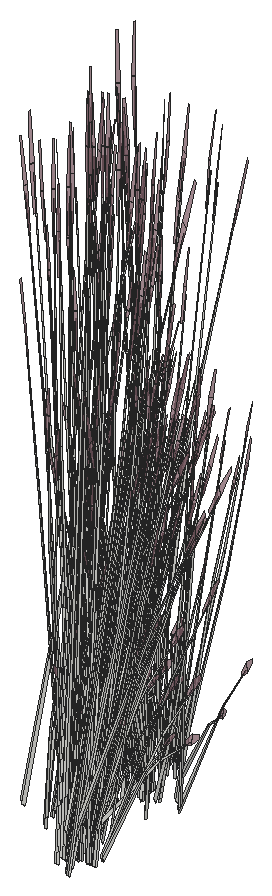
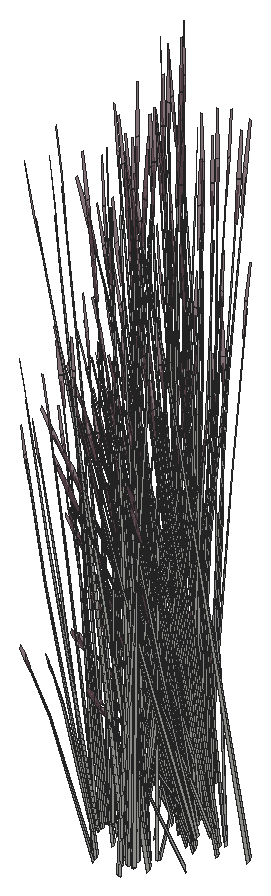
# SketchUp Ruby script. Lengths in inches.
U = 1.inch
M = Sketchup.active_model
def pt(a) = Geom::Point3d.new(a.map { |v| v * U })
def face(e, loops, mat)
  f = e.add_face(loops[0].map { |a| pt(a) })
  loops[1..].each { |l| e.add_face(l.map { |a| pt(a) }).erase! }
  f.material = f.back_material = mat if mat
  f
end
# faces: each face lists its corners as indices into pts; further lists are holes
def faces(e, pts, list, mat = nil) = list.each { |f| face(e, (f[0].is_a?(Array) ? f : [f]).map { |l| l.map { |i| pts[i] } }, mat) }
# xy, xz, yz: faces in a plane at the given z, y or x. An outline is a flat list of corners, or four numbers for a rectangle; further outlines are holes
def ring(l) = l.size == 4 ? [[l[0], l[1]], [l[2], l[1]], [l[2], l[3]], [l[0], l[3]]] : l.each_slice(2).to_a
def flat(e, list, mat, &to3) = list.each { |f| face(e, (f[0].is_a?(Array) ? f : [f]).map { |l| ring(l).map { |u, v| to3.(u, v) } }, mat) }
def xy(e, z, list, mat = nil) = flat(e, list, mat) { |x, y| [x, y, z] }
def xz(e, y, list, mat = nil) = flat(e, list, mat) { |x, z| [x, y, z] }
def yz(e, x, list, mat = nil) = flat(e, list, mat) { |y, z| [x, y, z] }
def lines(e, pts, list) = list.each { |a, b| e.add_line(pt(pts[a]), pt(pts[b])) }
# prism: a flat outline (further loops are holes) pulled along v
def prism(e, loops, v, mat = nil)
  f = face(e, loops, mat); d = Geom::Vector3d.new(v.map { |x| x * U })
  f.pushpull(f.normal.samedirection?(d) ? d.length : -d.length)
end
def box(e, o, s, mat = nil) = prism(e, [[o, [o[0] + s[0], o[1], o[2]], [o[0] + s[0], o[1] + s[1], o[2]], [o[0], o[1] + s[1], o[2]]]], [0, 0, s[2]], mat)
def at(x, y, z, deg = 0) = Geom::Transformation.translation(pt([x, y, z])) * Geom::Transformation.rotation(ORIGIN, Z_AXIS, deg.degrees)
def axes(o, x, y, z) = Geom::Transformation.new([*x, 0, *y, 0, *z, 0, *pt(o).to_a, 1])
def part(name) = M.definitions.add(name)
# library, detail: a bought-in or finely detailed component or shape, given as its bounding box
def library(name, o, s) = part(name).tap { |d| box(d.entities, o, s) }
def detail(e, o, s) = box(e.add_group.entities, o, s)
def put(e, d, t, mat = nil) = e.add_instance(d, t).tap { |i| i.material = mat if mat }
def group(e, t, mat = nil) = e.add_group.tap { |g| g.transformation = t; g.material = mat if mat }.entities
root = M.entities
M.materials.add("LightPink_Translucent").color = [144, 107, 117]
M.materials["LightPink_Translucent"].alpha = 0.75
c1 = part("blade")
p = [[2.15,0.21,22],[0,0.17,0],[0.09,0.45,0],[2.18,0.31,22],[2.29,0.31,22],[0.38,0.45,0],
  [2.48,0.24,33],[2.49,0.24,33],[2.48,0.22,33]]
faces(c1.entities,p,[[0,1,2,3],[4,5,2,3],[6,3,4,7],[8,0,3,6]])
c2 = part("seeds")
p = [[0.3,-0.1,1.38],[-0.01,-0.03,1.59],[-0.01,-0.03,0.03],[0.14,-0.07,-0.07],[0.29,-0.03,3],[0.15,0.01,3.11]]
faces(c2.entities,p,[[0,1,2,3],[1,0,4,5]],"LightPink_Translucent")
c3 = part("blade with seeds")
put(c3.entities,c1,at(0,0,0))
put(c3.entities,c2,axes([2.4,0.25,30.99],[1.5799,-0.05474,1.17369],[-0.12525,1.92788,0.29478],[-0.07173,-0.02425,1.56792]))
put(root,c3,axes([411.99,41.31,-7.78],[0.42502,0.15163,-0.32977],[-0.12396,0.44238,0.42575],[0.17112,-0.04056,0.81462]))
put(root,c3,axes([411.24,39.4,-10.12],[0.47863,0.27177,-0.46235],[-0.28609,0.48733,0],[0.10901,0.0619,1.46668]))
put(root,c3,axes([410.33,40.95,-9.95],[0.57217,0,0],[0,0.56272,0],[0,0,1.66132]))
put(root,c3,axes([410.49,39.63,-9.7],[-0.54955,0.14427,0.16428],[-0.1357,-0.53689,0.32672],[0.04901,0.07823,1.49371]))
put(root,c3,axes([410.83,40.76,-8.39],[-0.21212,0.01231,1.59586],[0.14072,-0.53355,0.12904],[0.3023,0.033,0.68222]))
put(root,c3,axes([411.1,39.6,-10.11],[0.12013,0.47362,-0.28847],[-0.47712,0.13449,0.28847],[0.09619,0.05462,1.29413]))
put(root,c3,axes([411.93,41.5,-7.6],[0.18783,0.37061,0.05988],[-0.34252,0.1814,0.47138],[0.15099,-0.03579,0.71878]))
put(root,c3,axes([410.14,40.66,-9.78],[-0.64638,-0.11452,0.45814],[0.13155,-0.64678,0.17978],[0.09446,0.06245,1.59061]))
put(root,c3,axes([411.89,41.36,-7.59],[-0.14449,0.4956,0.447],[-0.47502,-0.16947,0.36857],[0.1868,-0.02978,0.92496]))
put(root,c3,axes([409.63,42.26,-9.95],[-0.16686,-0.46861,0],[0.47648,-0.16411,0],[0,0,1.4375]))
put(root,c3,axes([409.31,41.81,-9.5625],[-0.09866,0.48509,0.13483],[-0.48202,-0.0842,-0.38503],[-0.08772,-0.04981,1.18024]))
put(root,c3,axes([410.25,42.19,-9.97],[0.53691,-0.18442,-0.17877],[0.18866,0.53125,0.00007],[0.05927,-0.02038,1.61933]))
put(root,c3,axes([410.4375,42.42,-9.7],[0.14774,-0.54019,0.16428],[0.54062,0.15287,0.32672],[-0.09339,0.00263,1.49371]))
put(root,c3,axes([410.32,41.19,-9.9375],[0.35699,0.35109,0],[-0.35699,0.35109,0],[0,0,1.57621]))
put(root,c3,axes([411.28,41.04,-9.7],[-0.40181,-0.39593,0.16428],[0.40492,-0.38402,0.32672],[-0.04438,0.08086,1.49371]))
put(root,c3,axes([410.54,40.4375,-10.08],[0.53199,0.08911,-0.58063],[-0.11226,0.54969,-0.15239],[0.15876,0.06661,1.28164]))
put(root,c3,axes([412.89,41.4,-9.42],[-0.31598,0.08973,1.06958],[0.14873,-0.37085,0.78586],[0.16763,0.02538,0.23558]))
put(root,c3,axes([405.58,44.46,-10.61],[-0.07655,-0.04282,1.6421],[-0.19662,-0.47839,-0.25086],[0.13264,-0.12982,0.2797]))
put(root,c3,axes([409.51,42.47,-9.95],[-0.51557,-0.24403,0],[0.24813,-0.50705,0],[0,0,1.51513]))
put(root,c3,axes([408.625,42.66,-9.69],[0.47863,0.27177,0.46235],[-0.28609,0.48733,0],[-0.10901,-0.0619,1.46668]))
put(root,c3,axes([410.3125,40.78,-9.47],[0.24813,-0.48978,0.41661],[0.51557,0.23571,-0.2005],[0,0.1129,1.33761]))
put(root,c3,axes([412.74,42.97,-7.62],[-0.04624,-0.04758,1.65179],[0.10116,-0.51007,-0.15608],[0.18215,-0.03259,0.29231]))
put(root,c3,axes([410.22,41.06,-9.87],[0,0.62861,-0.05249],[-0.63949,0,0],[0,0.01975,1.67027]))
put(root,c3,axes([410.26,40.61,-9.94],[0.30722,0.45622,-0.41661],[-0.46535,0.32126,0.2005],[0.09942,0.05645,1.33761]))
put(root,c3,axes([412.34,42.54,-8.34],[-0.09788,-0.45691,-0.03251],[0.46264,-0.10504,-0.14742],[0.09661,0.02897,0.48626]))
put(root,c3,axes([411.14,42.53,-7.3125],[0.02738,-0.55277,-0.11324],[0.51847,0.01511,-0.62851],[0.19968,0.0384,0.95501]))
put(root,c3,axes([405.58,45.81,-7.36],[0.26714,-0.42887,-0.66157],[0.46811,0.30479,0.07984],[0.1595,-0.15539,0.93586]))
put(root,c3,axes([405.5625,45.61,-7.64],[-0.13138,-0.49631,-0.47583],[0.49754,-0.08682,-0.36857],[0.14258,-0.13331,0.91046]))
put(root,c3,axes([411.61,41.05,-9.69],[0,-0.54355,0.46235],[0.57217,0,0],[0,0.1238,1.46668]))
put(root,c3,axes([410.18,41.46,-9.47],[0.55535,-0.03355,0.41661],[0.05022,0.55698,-0.2005],[-0.09942,0.05645,1.33761]))
put(root,c3,axes([410.53,40.89,-9.5625],[0.47648,-0.15851,0.13483],[0.16686,0.45265,-0.38503],[0,0.09962,1.18024]))
put(root,c3,axes([411.0625,42.3125,-7.3],[-0.29098,-0.34031,0.32977],[0.33226,-0.32215,-0.42575],[0.16881,0.04902,0.81462]))
put(root,c3,axes([405.8,45.96,-7.3125],[-0.47307,-0.29971,-0.11324],[0.27254,-0.43404,-0.62851],[0.13365,-0.15087,0.95501]))
put(root,c3,axes([412.3,41.99,-9.59],[-0.12317,-0.13368,1.33163],[0.16025,-0.44223,-0.28638],[0.24919,0.05991,0.56934]))
put(root,c3,axes([410.1,42.48,-9.95],[0.51557,0.24403,0],[-0.24813,0.50705,0],[0,0,1.62917]))
put(root,c3,axes([405.96,45.41,-9.59],[-0.1827,-0.0161,1.33163],[-0.18717,-0.43188,-0.28638],[0.22444,-0.12218,0.56934]))
put(root,c3,axes([406.96,45.83,-7.62],[-0.0668,-0.00413,1.65179],[-0.27738,-0.44233,-0.15608],[0.11139,-0.14544,0.29231]))
put(root,c3,axes([411.59,42.2,-7.61],[0.10971,-0.00919,1.62908],[0.30091,-0.42228,-0.25764],[0.19514,0.05574,0.13065]))
put(root,c3,axes([410.3,43.02,-9.96],[-0.31576,-0.54657,-0.04789],[0.53494,-0.30375,0.48057],[-0.13182,0.05204,1.52373]))
put(root,c3,axes([410.1875,41.7,-9.5625],[0.37783,0.32657,0.13483],[-0.31516,0.36844,-0.38503],[-0.08772,0.04981,1.18024]))
put(root,c3,axes([406.17,44.62,-9.42],[-0.17034,0.27669,1.06958],[-0.14642,-0.37174,0.78586],[0.14069,-0.09315,0.23558]))
put(root,c3,axes([411.17,42.26,-7.36],[0.51122,0.01309,-0.66157],[-0.03434,0.5511,0.07984],[0.21658,0.05816,0.93586]))
put(root,c3,axes([405.93,45.66,-7.78],[0.44516,-0.07768,-0.32977],[0.11755,0.44407,0.42575],[0.12757,-0.11927,0.81462]))
put(root,c3,axes([410.59,42.7,-9.69],[0.47863,-0.27177,0.46235],[0.28609,0.48733,0],[-0.10901,0.0619,1.46668]))
put(root,c3,axes([409.91,42.28,-9.87],[0.22235,0.62444,-0.05599],[-0.63531,0.21881,0],[0.00776,0.02181,1.60327]))
put(root,c3,axes([410.16,42.95,-10.11],[-0.47712,-0.13449,-0.28847],[0.12013,-0.47362,0.28847],[-0.09619,0.05462,1.29413]))
put(root,c3,axes([412,41.14,-9.79],[0.63949,0,0],[0,0.60749,-0.48057],[0,0.13836,1.52448]))
put(root,c3,axes([411.75,41.46,-9.95],[-0.63917,-0.00435,-0.04634],[0,-0.60749,0.46507],[-0.02009,0.13829,1.47457]))
put(root,c3,axes([410.36,40.93,-9.52],[0.57594,0.25935,-0.27094],[-0.27732,0.5474,-0.46562],[0.0181,0.1344,1.4872]))
put(root,c3,axes([411.47,42.49,-7.78],[0.29098,0.34031,-0.32977],[-0.33226,0.32215,0.42575],[0.16881,0.04902,0.81462]))
put(root,c3,axes([411.61,41.54,-10.11],[-0.35699,0.33913,-0.28847],[-0.35699,-0.33913,0.28847],[0,0.10923,1.29413]))
put(root,c3,axes([410.07,41.58,-9.52],[0.05959,0.62022,-0.27094],[-0.62068,0.0375,-0.46562],[-0.1093,0.08261,1.4872]))
put(root,c3,axes([411.33,42.62,-7.6],[-0.02575,0.41332,0.05988],[-0.38885,-0.01133,0.47138],[0.14895,0.04325,0.71878]))
put(root,c3,axes([410.3,41.34,-9.94],[-0.24813,0.48978,-0.41661],[-0.51557,-0.23571,0.2005],[0,0.1129,1.33761]))
put(root,c3,axes([411.36,42.49,-7.59],[-0.37709,0.35815,0.447],[-0.32522,-0.38035,0.36857],[0.17692,0.06607,0.92496]))
put(root,c3,axes([405.97,45.85,-7.6],[0.35109,0.22859,0.05988],[-0.2044,0.32553,0.47138],[0.11256,-0.10524,0.71878]))
put(root,c3,axes([405.87,45.75,-7.59],[0.12683,0.50025,0.447],[-0.49754,0.08682,0.36857],[0.14663,-0.11765,0.92496]))
put(root,c3,axes([407.21,46.36,-7.61],[0.07097,-0.08279,1.62908],[-0.09083,-0.50786,-0.25764],[0.17806,-0.09629,0.13065]))
put(root,c3,axes([410.16,42.9,-7.3],[-0.07899,-0.43781,0.32977],[0.45153,-0.11561,-0.42575],[0.12128,0.12546,0.81462]))
put(root,c3,axes([410.31,42.74,-9.83],[0.64025,0.17667,0.2864],[-0.16018,0.63149,-0.33981],[-0.10597,0.07904,1.53541]))
put(root,c3,axes([410.27,43.17,-10.12],[-0.47863,0.27177,-0.46235],[-0.28609,-0.48733,0],[-0.10901,0.0619,1.46668]))
put(root,c3,axes([411.86,41.56,-10.12],[0,0.54355,-0.46235],[-0.57217,0,0],[0,0.1238,1.46668]))
put(root,c3,axes([410.43,41.62,-8.39],[-0.18996,-0.09365,1.59586],[0.39312,-0.39287,0.12904],[0.24502,0.17723,0.68222]))
put(root,c3,axes([410.47,40.39,-7.83],[-0.44191,-0.28242,1.28769],[0.46662,-0.43971,0.5556],[0.14258,0.26499,1.24467]))
put(root,c3,axes([411.13,42.68,-9.42],[-0.28795,-0.15629,1.06958],[0.37181,-0.1588,0.78586],[0.10029,0.13452,0.23558]))
put(root,c3,axes([410.12,43.13,-7.3125],[0.30474,-0.46525,-0.11324],[0.44133,0.26804,-0.62851],[0.15341,0.13145,0.95501]))
put(root,c3,axes([409.05,49.32,-9.59],[-0.14537,0.11002,1.33163],[-0.43536,-0.19256,-0.28638],[0.0807,-0.23948,0.56934]))
put(root,c3,axes([408.11,42.5,-7.3],[0.34603,-0.28618,0.32977],[0.32756,0.32677,-0.42575],[-0.04984,0.16603,0.81462]))
put(root,c3,axes([410.7,43.08,-9.79],[0.31974,0.54466,0],[-0.53494,0.30375,-0.48057],[-0.12184,0.06918,1.52448]))
put(root,c3,axes([405.82,47.13,-7.3125],[-0.25732,-0.49218,-0.11324],[0.45669,-0.24187,-0.62851],[0.19245,-0.06494,0.95501]))
put(root,c3,axes([405.79,46.71,-7.64],[0.13855,-0.49442,-0.47583],[0.47502,0.16947,-0.36857],[0.19125,-0.04534,0.91046]))
put(root,c3,axes([405.04,44.7,-9.79],[0.31974,-0.54466,0],[0.53494,0.30375,-0.48057],[0.12184,0.06918,1.52448]))
put(root,c3,axes([409.72,43.52,-7.62],[0.00151,-0.06581,1.65179],[0.43826,-0.29033,-0.15608],[0.15223,0.10363,0.29231]))
put(root,c3,axes([411.21,43.26,-10.61],[0.03726,-0.07847,1.6421],[0.46909,-0.23111,-0.25086],[0.14221,0.11962,0.2797]))
put(root,c3,axes([410.43,40.93,-9.35],[-0.01397,-0.51177,1.31553],[0.63227,0.13266,0.557],[-0.14954,0.28003,1.24175]))
put(root,c3,axes([410.59,41.48,-10.05],[0.18752,0.49766,-0.6445],[-0.54017,0.17923,-0.16915],[0.02073,0.16852,1.42262]))
put(root,c3,axes([410.48,42.9,-7.64],[0.50465,-0.12921,-0.47583],[0.08828,0.48932,-0.36857],[0.13555,0.14022,0.91046]))
put(root,c3,axes([407.97,48.72,-10.61],[-0.08578,0.01958,1.6421],[-0.47437,-0.22044,-0.25086],[0.00796,-0.18387,0.2797]))
put(root,c3,axes([406.3,46.85,-10.15],[-0.32938,0.06523,1.31842],[-0.05243,-0.51922,0.07547],[0.2307,-0.07859,0.75023]))
put(root,c3,axes([406.9,46.39,-9.89],[-0.31706,-0.34757,-0.06041],[0.34725,-0.31847,-0.27392],[0.09839,-0.02242,0.90349]))
put(root,c3,axes([409.08,42.97,-7.3],[0.15418,-0.41799,0.32977],[0.44981,0.12192,-0.42575],[0.04124,0.16829,0.81462]))
put(root,c3,axes([409.4,50.14,-7.36],[0.01331,-0.50278,-0.66157],[0.56035,0.03377,0.07984],[0.05914,-0.213,0.93586]))
put(root,c3,axes([411.18,43.4,-9.52],[-0.32795,-0.01705,0.97832],[0.21658,-0.36206,0.54015],[0.12956,0.12863,0.76741]))
put(root,c3,axes([405.7,46.89,-7.36],[0.44939,-0.24006,-0.66157],[0.25044,0.49415,0.07984],[0.21713,-0.05613,0.93586]))
put(root,c3,axes([410.18,49.35,-7.61],[-0.00494,-0.10818,1.62908],[-0.41695,-0.31265,-0.25764],[0.06446,-0.18952,0.13065]))
put(root,c3,axes([408.43,49.33,-7.78],[0.15418,-0.41799,-0.32977],[0.44981,0.12192,0.42575],[-0.04124,-0.16829,0.81462]))
put(root,c3,axes([408.77,49.88,-8.39],[-0.09522,0.18683,1.59586],[-0.39947,-0.38663,0.12904],[0.18021,-0.24097,0.68222]))
put(root,c3,axes([410.07,48.96,-7.62],[-0.05194,0.04152,1.65179],[-0.50886,-0.14007,-0.15608],[-0.01842,-0.18118,0.29231]))
put(root,c3,axes([410.23,43.3,-7.6],[-0.23243,0.34529,0.05988],[-0.331,-0.20103,0.47138],[0.10701,0.1107,0.71878]))
put(root,c3,axes([409.6875,44.46,-6.74],[0.35341,-0.31182,-0.06041],[0.32382,0.34152,-0.27392],[0.0228,0.09677,0.90349]))
put(root,c3,axes([410.33,43.2,-7.59],[-0.50866,0.12474,0.447],[-0.08828,-0.48932,0.36857],[0.11963,0.14421,0.92496]))
put(root,c3,axes([408.51,48.45,-9.42],[0.06561,0.31695,1.06958],[-0.36394,-0.17555,0.78586],[0.03916,-0.16229,0.23558]))
put(root,c3,axes([405.64,46.98,-7.3],[-0.42502,-0.15163,0.32977],[0.12396,-0.44238,-0.42575],[0.17112,-0.04056,0.81462]))
put(root,c3,axes([409.29,49.97,-7.64],[-0.3661,-0.36521,-0.47583],[0.38674,-0.31985,-0.36857],[0.0557,-0.18556,0.91046]))
put(root,c3,axes([402.73,45.66,-10.52],[-0.50338,0.21762,1.20058],[-0.16022,-0.62439,0.4665],[0.30911,0.01039,1.36553]))
put(root,c3,axes([410.11,42.52,-9.59],[0.00902,-0.18018,1.33163],[0.43127,-0.20126,-0.28638],[0.13313,0.21566,0.56934]))
put(root,c3,axes([406.66,46.51,-10.61],[-0.02673,-0.08252,1.6421],[0.18538,-0.48271,-0.25086],[0.187,-0.00694,0.2797]))
put(root,c3,axes([408.94,43.35,-7.6],[-0.37684,0.18473,0.05988],[-0.18445,-0.33686,0.47138],[0.03639,0.14849,0.71878]))
put(root,c3,axes([407.89,42.58,-6.97],[0.56206,0.02693,-0.12569],[-0.01536,0.50991,-0.69765],[-0.03904,0.19638,1.06006]))
put(root,c3,axes([408.93,43.15,-7.3125],[0.50045,-0.25306,-0.11324],[0.24593,0.44915,-0.62851],[0.06603,0.18927,0.95501]))
put(root,c3,axes([409.08,43.32,-7.28],[-0.50393,-0.1421,0.49617],[0.17232,-0.46717,0.40911],[0.03028,0.18372,1.0267]))
put(root,c3,axes([408.49,49.43,-7.59],[0.50393,0.1421,0.447],[-0.17232,0.46717,0.36857],[-0.03028,-0.18372,0.92496]))
put(root,c3,axes([409.67,50.16,-7.3125],[-0.56206,-0.02693,-0.11324],[0.01536,-0.50991,-0.62851],[0.03904,-0.19638,0.95501]))
put(root,c3,axes([409.63,49.84,-7.78],[0.34603,-0.28618,-0.32977],[0.32756,0.32677,0.42575],[0.04984,-0.16603,0.81462]))
put(root,c3,axes([408.62,49.39,-7.6],[0.37684,-0.18473,0.05988],[0.18445,0.33686,0.47138],[-0.03639,-0.14849,0.71878]))
put(root,c3,axes([406.09,46.93,-7.78],[0.42502,0.15163,-0.32977],[-0.12396,0.44238,0.42575],[0.17112,-0.04056,0.81462]))
put(root,c3,axes([409.02,43.25,-10.61],[0.08277,-0.02958,1.6421],[0.49786,0.16279,-0.25086],[0.01456,0.18348,0.2797]))
put(root,c3,axes([405.33,45.02,-10.12],[0.47863,0.27177,-0.46235],[-0.28609,0.48733,0],[0.10901,0.0619,1.46668]))
put(root,c3,axes([408.28,42.77,-7.34],[0.3661,0.36521,-0.52818],[-0.38674,0.31985,-0.40911],[-0.0557,0.18556,1.01061]))
put(root,c3,axes([407.88,43.32,-9.37],[0.46459,-0.09625,0.0606],[0.10681,0.38778,-0.80367],[-0.02945,0.1963,0.72038]))
put(root,c3,axes([409.36,43.125,-7.64],[0.50273,0.13626,-0.47583],[-0.17232,0.46717,-0.36857],[0.0461,0.18809,0.91046]))
put(root,c3,axes([409.65,42.16,-8.39],[-0.1169,-0.17452,1.59586],[0.54019,-0.14692,0.12904],[0.12209,0.27397,0.68222]))
put(root,c3,axes([404.93,46.39,-8.39],[-0.21212,0.01231,1.59586],[0.14072,-0.53355,0.12904],[0.3023,0.033,0.68222]))
put(root,c3,axes([409.13,43.41,-7.78],[-0.15418,0.41799,-0.32977],[-0.44981,-0.12192,0.42575],[0.04124,0.16829,0.81462]))
put(root,c3,axes([406.02,47.12,-7.6],[0.18783,0.37061,0.05988],[-0.34252,0.1814,0.47138],[0.15099,-0.03579,0.71878]))
put(root,c3,axes([405.99,46.99,-7.59],[-0.14449,0.4956,0.447],[-0.47502,-0.16947,0.36857],[0.1868,-0.02978,0.92496]))
put(root,c3,axes([410.07,49.66,-10.61],[-0.07655,-0.04282,1.6421],[-0.19662,-0.47839,-0.25086],[0.13264,-0.12982,0.2797]))
put(root,c3,axes([408.48,49.77,-7.3],[-0.15418,0.41799,0.32977],[-0.44981,-0.12192,-0.42575],[-0.04124,-0.16829,0.81462]))
put(root,c3,axes([408.69,42.25,-8.39],[-0.01252,-0.20862,1.59586],[0.54251,0.1384,0.12904],[-0.03356,0.2973,0.68222]))
put(root,c3,axes([409.63,49.95,-7.59],[0.36417,0.37086,0.447],[-0.38674,0.31985,0.36857],[0.06718,-0.174,0.92496]))
put(root,c3,axes([409.77,49.98,-7.6],[0.42027,0.02533,0.05988],[-0.01152,0.38243,0.47138],[0.04398,-0.14649,0.71878]))
put(root,c3,axes([404.64,46.0625,-10.08],[0.53199,0.08911,-0.58063],[-0.11226,0.54969,-0.15239],[0.15876,0.06661,1.28164]))
put(root,c3,axes([406.99,47.02,-9.42],[-0.31598,0.08973,1.06958],[0.14873,-0.37085,0.78586],[0.16763,0.02538,0.23558]))
put(root,c3,axes([409.45,50.24,-7.3],[-0.34603,0.28618,0.32977],[-0.32756,-0.32677,-0.42575],[0.04984,-0.16603,0.81462]))
put(root,c3,axes([409.18,43.04,-7.36],[0.24409,0.44196,-0.66157],[-0.50245,0.2463,0.07984],[0.05708,0.21354,0.93586]))
put(root,c3,axes([410.0625,51.01,-7.36],[0.26714,-0.42887,-0.66157],[0.46811,0.30479,0.07984],[0.1595,-0.15539,0.93586]))
put(root,c3,axes([407.18,49.76,-9.79],[-0.31974,-0.54466,0],[0.53494,-0.30375,-0.48057],[0.12184,-0.06918,1.52448]))
put(root,c3,axes([410.05,50.8125,-7.64],[-0.13138,-0.49631,-0.47583],[0.49754,-0.08682,-0.36857],[0.14258,-0.13331,0.91046]))
put(root,c3,axes([408.8125,44.15,-7.61],[0.06483,0.08753,1.62908],[0.52315,0.03439,-0.25764],[0.05261,0.19303,0.13065]))
put(root,c3,axes([406.84,48.59,-7.62],[-0.04624,-0.04758,1.65179],[0.10116,-0.51007,-0.15608],[0.18215,-0.03259,0.29231]))
put(root,c3,axes([410.29,51.17,-7.3125],[-0.47307,-0.29971,-0.11324],[0.27254,-0.43404,-0.62851],[0.13365,-0.15087,0.95501]))
put(root,c3,axes([406.4375,48.17,-8.34],[-0.09788,-0.45691,-0.03251],[0.46264,-0.10504,-0.14742],[0.09661,0.02897,0.48626]))
put(root,c3,axes([405.24,48.15,-7.3125],[0.02738,-0.55277,-0.11324],[0.51847,0.01511,-0.62851],[0.19968,0.0384,0.95501]))
put(root,c3,axes([407.61,49.68,-10.12],[0.47863,-0.27177,-0.46235],[0.28609,0.48733,0],[0.10901,-0.0619,1.46668]))
put(root,c3,axes([405.16,47.9375,-7.3],[-0.29098,-0.34031,0.32977],[0.33226,-0.32215,-0.42575],[0.16881,0.04902,0.81462]))
put(root,c3,axes([410.45,50.62,-9.59],[-0.1827,-0.0161,1.33163],[-0.18717,-0.43188,-0.28638],[0.22444,-0.12218,0.56934]))
put(root,c3,axes([411.45,51.04,-7.62],[-0.0668,-0.00413,1.65179],[-0.27738,-0.44233,-0.15608],[0.11139,-0.14544,0.29231]))
put(root,c3,axes([407.97,43.3125,-8.87],[0.01124,-0.2806,1.43727],[0.50537,0.14821,0.19862],[-0.04379,0.29905,0.67868]))
put(root,c3,axes([406.39,47.62,-9.59],[-0.12317,-0.13368,1.33163],[0.16025,-0.44223,-0.28638],[0.24919,0.05991,0.56934]))
put(root,c3,axes([408.18,50.79,-10.08],[0.34446,-0.40855,-0.58063],[0.42791,0.37046,-0.15239],[0.13803,-0.10191,1.28164]))
put(root,c3,axes([410.66,49.82,-9.42],[-0.17034,0.27669,1.06958],[-0.14642,-0.37174,0.78586],[0.14069,-0.09315,0.23558]))
put(root,c3,axes([410.42,50.86,-7.78],[0.44516,-0.07768,-0.32977],[0.11755,0.44407,0.42575],[0.12757,-0.11927,0.81462]))
put(root,c3,axes([405.69,47.82,-7.61],[0.10971,-0.00919,1.62908],[0.30091,-0.42228,-0.25764],[0.19514,0.05574,0.13065]))
put(root,c3,axes([407.58,51.51,-9.94],[0.24813,-0.48978,-0.41661],[0.51557,0.23571,0.2005],[0,-0.1129,1.33761]))
put(root,c3,axes([407.8,51.27,-9.52],[-0.05959,-0.62022,-0.27094],[0.62068,-0.0375,-0.46562],[0.1093,-0.08261,1.4872]))
put(root,c3,axes([410.05,51.125,-7.3],[-0.44516,0.07768,0.32977],[-0.11755,-0.44407,-0.42575],[0.12757,-0.11927,0.81462]))
put(root,c3,axes([405.26,47.89,-7.36],[0.51122,0.01309,-0.66157],[-0.03434,0.5511,0.07984],[0.21658,0.05816,0.93586]))
put(root,c3,axes([407.72,49.89,-10.11],[0.47712,0.13449,-0.28847],[-0.12013,0.47362,0.28847],[0.09619,-0.05462,1.29413]))
put(root,c3,axes([410.46,51.06,-7.6],[0.35109,0.22859,0.05988],[-0.2044,0.32553,0.47138],[0.11256,-0.10524,0.71878]))
put(root,c3,axes([405.57,48.12,-7.78],[0.29098,0.34031,-0.32977],[-0.33226,0.32215,0.42575],[0.16881,0.04902,0.81462]))
put(root,c3,axes([410.36,50.96,-7.59],[0.12683,0.50025,0.447],[-0.49754,0.08682,0.36857],[0.14663,-0.11765,0.92496]))
put(root,c3,axes([411.7,51.5625,-7.61],[0.07097,-0.08279,1.62908],[-0.09083,-0.50786,-0.25764],[0.17806,-0.09629,0.13065]))
put(root,c3,axes([405.42,48.25,-7.6],[-0.02575,0.41332,0.05988],[-0.38885,-0.01133,0.47138],[0.14895,0.04325,0.71878]))
put(root,c3,axes([405.46,48.11,-7.59],[-0.37709,0.35815,0.447],[-0.32522,-0.38035,0.36857],[0.17692,0.06607,0.92496]))
put(root,c3,axes([407.89,51.75,-9.73],[0.57623,0.26344,0.22409],[-0.27732,0.5474,0.46562],[0,-0.12618,1.49497]))
put(root,c3,axes([404.53,47.24,-8.39],[-0.18996,-0.09365,1.59586],[0.39312,-0.39287,0.12904],[0.24502,0.17723,0.68222]))
put(root,c3,axes([407.7,51.39,-9.47],[-0.55535,0.03355,0.41661],[-0.05022,-0.55698,-0.2005],[0.09942,-0.05645,1.33761]))
put(root,c3,axes([410.3,52.34,-7.3125],[-0.25732,-0.49218,-0.11324],[0.45669,-0.24187,-0.62851],[0.19245,-0.06494,0.95501]))
put(root,c3,axes([410.28,51.91,-7.64],[0.13855,-0.49442,-0.47583],[0.47502,0.16947,-0.36857],[0.19125,-0.04534,0.91046]))
put(root,c3,axes([409.53,49.9,-9.79],[0.31974,-0.54466,0],[0.53494,0.30375,-0.48057],[0.12184,0.06918,1.52448]))
put(root,c3,axes([407.68,51.59,-9.8],[0.22235,0.6078,0.42607],[-0.63531,0.21135,0.16719],[0.00776,-0.11168,1.47927]))
put(root,c3,axes([404.22,48.76,-7.3125],[0.30474,-0.46525,-0.11324],[0.44133,0.26804,-0.62851],[0.15341,0.13145,0.95501]))
put(root,c3,axes([410.79,52.05,-10.15],[-0.32938,0.06523,1.31842],[-0.05243,-0.51922,0.07547],[0.2307,-0.07859,0.75023]))
put(root,c3,axes([411.39,51.59,-9.89],[-0.31706,-0.34757,-0.06041],[0.34725,-0.31847,-0.27392],[0.09839,-0.02242,0.90349]))
put(root,c3,axes([408.48,51.64,-9.95],[0,-0.62892,0],[0.63949,0,0],[0,0,1.6711]))
put(root,c3,axes([409.26,50.18,-9.69],[-0.47863,-0.27177,0.46235],[0.28609,-0.48733,0],[0.10901,0.0619,1.46668]))
put(root,c3,axes([410.19,52.09,-7.36],[0.44939,-0.24006,-0.66157],[0.25044,0.49415,0.07984],[0.21713,-0.05613,0.93586]))
put(root,c3,axes([405.3125,48.89,-10.61],[0.03726,-0.07847,1.6421],[0.46909,-0.23111,-0.25086],[0.14221,0.11962,0.2797]))
put(root,c3,axes([408.18,51.24,-9.8],[-0.42403,0.49328,0.42607],[-0.50377,-0.43543,0.16719],[0.10223,-0.04923,1.47927]))
put(root,c3,axes([404.58,48.52,-7.64],[0.50465,-0.12921,-0.47583],[0.08828,0.48932,-0.36857],[0.13555,0.14022,0.91046]))
put(root,c3,axes([408.64,52.125,-9.86],[-0.47569,-0.46784,-0.05709],[0.47598,-0.46812,0],[-0.01661,-0.01634,1.63492]))
put(root,c3,axes([407.44,50.43,-9.7],[-0.14774,0.54019,0.16428],[-0.54062,-0.15287,0.32672],[0.09339,-0.00263,1.49371]))
put(root,c3,axes([410.125,52.1875,-7.3],[-0.42502,-0.15163,0.32977],[0.12396,-0.44238,-0.42575],[0.17112,-0.04056,0.81462]))
put(root,c3,axes([407.22,50.87,-10.52],[-0.50338,0.21762,1.20058],[-0.16022,-0.62439,0.4665],[0.30911,0.01039,1.36553]))
put(root,c3,axes([408.57,51.03,-9.5625],[0.09866,-0.48509,0.13483],[0.48202,0.0842,-0.38503],[0.08772,0.04981,1.18024]))
put(root,c3,axes([411.15,51.71,-10.61],[-0.02673,-0.08252,1.6421],[0.18538,-0.48271,-0.25086],[0.187,-0.00694,0.2797]))
put(root,c3,axes([408.36,51.16,-9.47],[-0.30722,-0.45622,0.41661],[0.46535,-0.32126,-0.2005],[0.09942,0.05645,1.33761]))
put(root,c3,axes([407.39,53.22,-9.7],[0.54955,-0.14427,0.16428],[0.1357,0.53689,0.32672],[-0.04901,-0.07823,1.49371]))
put(root,c3,axes([408.52,51.1875,-9.52],[0.51635,-0.36087,-0.27094],[0.34336,0.5099,-0.46562],[0.1274,0.05178,1.4872]))
put(root,c3,axes([410.57,52.14,-7.78],[0.42502,0.15163,-0.32977],[-0.12396,0.44238,0.42575],[0.17112,-0.04056,0.81462]))
